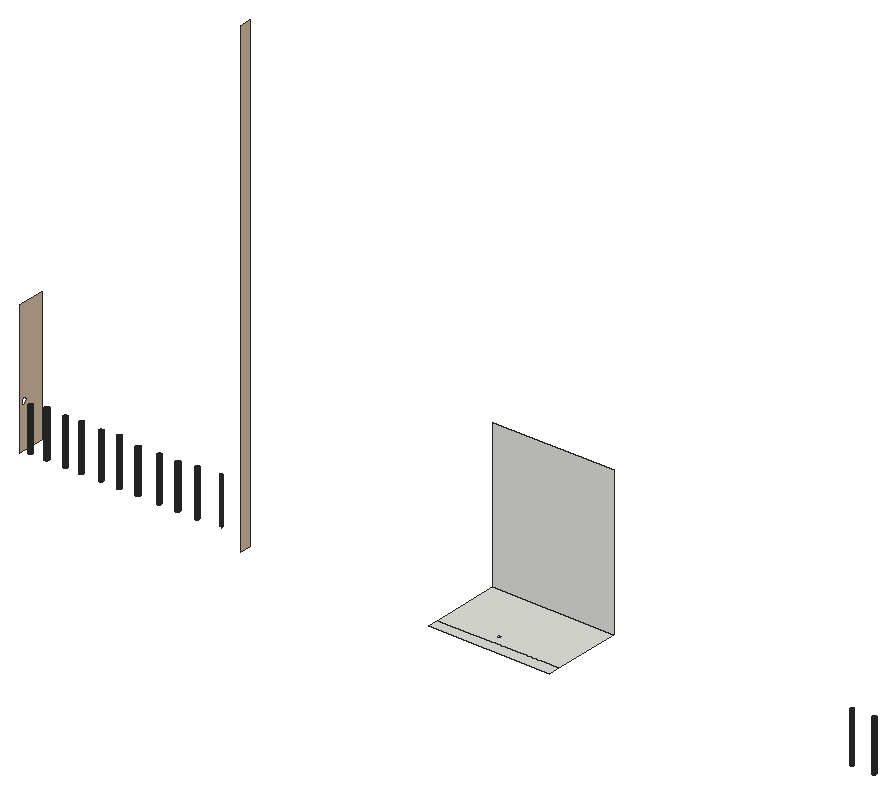
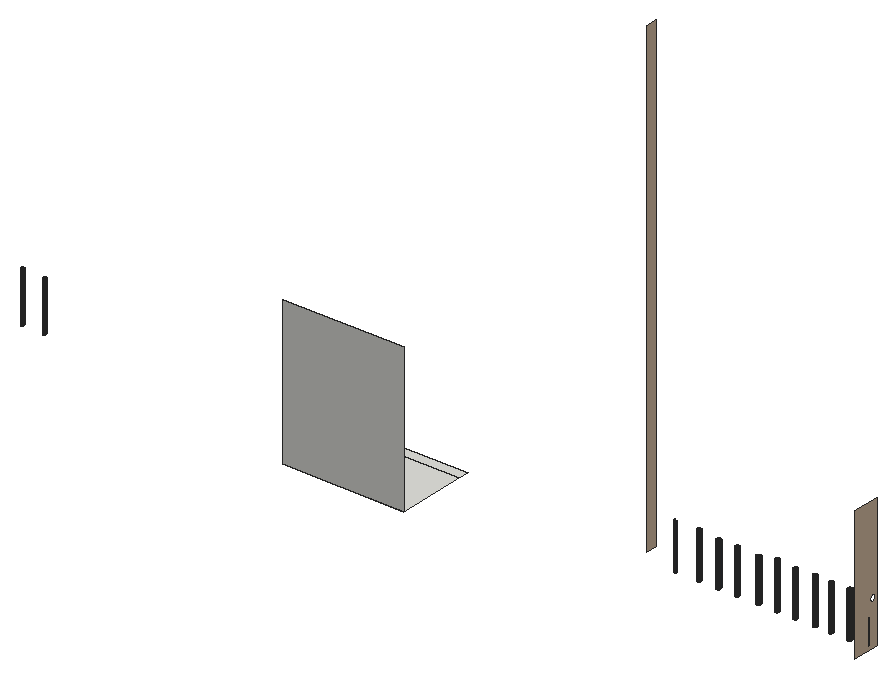
# SketchUp Ruby script. Lengths in inches.
U = 1.inch
M = Sketchup.active_model
def pt(a) = Geom::Point3d.new(a.map { |v| v * U })
def face(e, loops, mat)
  f = e.add_face(loops[0].map { |a| pt(a) })
  loops[1..].each { |l| e.add_face(l.map { |a| pt(a) }).erase! }
  f.material = f.back_material = mat if mat
  f
end
# faces: each face lists its corners as indices into pts; further lists are holes
def faces(e, pts, list, mat = nil) = list.each { |f| face(e, (f[0].is_a?(Array) ? f : [f]).map { |l| l.map { |i| pts[i] } }, mat) }
# xy, xz, yz: faces in a plane at the given z, y or x. An outline is a flat list of corners, or four numbers for a rectangle; further outlines are holes
def ring(l) = l.size == 4 ? [[l[0], l[1]], [l[2], l[1]], [l[2], l[3]], [l[0], l[3]]] : l.each_slice(2).to_a
def flat(e, list, mat, &to3) = list.each { |f| face(e, (f[0].is_a?(Array) ? f : [f]).map { |l| ring(l).map { |u, v| to3.(u, v) } }, mat) }
def xy(e, z, list, mat = nil) = flat(e, list, mat) { |x, y| [x, y, z] }
def xz(e, y, list, mat = nil) = flat(e, list, mat) { |x, z| [x, y, z] }
def yz(e, x, list, mat = nil) = flat(e, list, mat) { |y, z| [x, y, z] }
def lines(e, pts, list) = list.each { |a, b| e.add_line(pt(pts[a]), pt(pts[b])) }
# prism: a flat outline (further loops are holes) pulled along v
def prism(e, loops, v, mat = nil)
  f = face(e, loops, mat); d = Geom::Vector3d.new(v.map { |x| x * U })
  f.pushpull(f.normal.samedirection?(d) ? d.length : -d.length)
end
def box(e, o, s, mat = nil) = prism(e, [[o, [o[0] + s[0], o[1], o[2]], [o[0] + s[0], o[1] + s[1], o[2]], [o[0], o[1] + s[1], o[2]]]], [0, 0, s[2]], mat)
def at(x, y, z, deg = 0) = Geom::Transformation.translation(pt([x, y, z])) * Geom::Transformation.rotation(ORIGIN, Z_AXIS, deg.degrees)
def axes(o, x, y, z) = Geom::Transformation.new([*x, 0, *y, 0, *z, 0, *pt(o).to_a, 1])
def part(name) = M.definitions.add(name)
# library, detail: a bought-in or finely detailed component or shape, given as its bounding box
def library(name, o, s) = part(name).tap { |d| box(d.entities, o, s) }
def detail(e, o, s) = box(e.add_group.entities, o, s)
def put(e, d, t, mat = nil) = e.add_instance(d, t).tap { |i| i.material = mat if mat }
def group(e, t, mat = nil) = e.add_group.tap { |g| g.transformation = t; g.material = mat if mat }.entities
root = M.entities
M.materials.add("[Formica Laminate Dark]").color = [50, 53, 60]
M.materials.add("[Formica Laminate Light]").color = [213, 189, 164]
xy(root,261,[[351.88,110.07,450.54,119.07],[[351.88,119.07,450.54,174.4375],[395.34,125.42,394.9,125.48,394.49,125.65,394.14,125.92,393.875,126.27,393.71,126.67,393.65,127.11,393.71,127.55,393.875,127.95,394.14,128.3,394.49,128.57,394.9,128.74,395.34,128.8,395.77,128.74,396.18,128.57,396.53,128.3,396.8,127.95,396.97,127.55,397.02,127.11,396.97,126.67,396.8,126.27,396.53,125.92,396.18,125.65,395.77,125.48]],[674.41,135.92,674.07,135.96,673.75,136.09,673.48,136.3,673.27,136.57,673.14,136.89,673.1,137.23,673.14,137.57,673.27,137.88,673.48,138.16,673.75,138.36,674.07,138.5,674.41,138.54,674.75,138.5,675.07,138.36,675.34,138.16,675.55,137.88,675.68,137.57,675.72,137.23,675.68,136.89,675.55,136.57,675.34,136.3,675.07,136.09,674.75,135.96],[692.47,135.92,692.13,135.96,691.82,136.09,691.55,136.3,691.34,136.57,691.21,136.89,691.16,137.23,691.21,137.57,691.34,137.88,691.55,138.16,691.82,138.36,692.13,138.5,692.47,138.54,692.8125,138.5,693.13,138.36,693.4,138.16,693.61,137.88,693.74,137.57,693.79,137.23,693.74,136.89,693.61,136.57,693.4,136.3,693.13,136.09,692.8125,135.96]])
xz(root,174.4375,[[351.88,261,450.54,381]])
yz(root,9,[[[122.79,261,144.21,369],[126.49,294.81,125.8,294.9,125.15,295.17,124.59,295.59,124.17,296.15,123.9,296.8,123.81,297.49,123.9,298.1875,124.17,298.84,124.59,299.39,125.15,299.82,125.8,300.09,126.49,300.18,127.1875,300.09,127.84,299.82,128.39,299.39,128.82,298.84,129.09,298.1875,129.18,297.49,129.09,296.8,128.82,296.15,128.39,295.59,127.84,295.17,127.1875,294.9]]],"[Formica Laminate Light]")
yz(root,198.57,[[110.07,261,119.07,645]],"[Formica Laminate Light]")
p = [[13.4,125.48,261],[13.84,125.42,261],[13.84,125.42,295.875],[13.4,125.48,295.875],[14.27,125.48,261],[14.27,125.48,295.875],
  [26.65,125.48,261],[27.09,125.42,261],[27.09,125.42,298.1875],[26.65,125.48,298.1875],[27.52,125.48,261],[27.52,125.48,298.1875],
  [41.96,125.48,261],[42.4,125.42,261],[42.4,125.42,297.49],[41.96,125.48,297.49],[42.84,125.48,261],[42.84,125.48,297.49],
  [54.96,125.48,261],[55.4,125.42,261],[55.4,125.42,298.1875],[54.96,125.48,298.1875],[55.84,125.48,261],[55.84,125.48,298.1875],
  [70.84,125.48,261],[71.27,125.42,261],[71.27,125.42,297.375],[70.84,125.48,297.375],[71.71,125.48,261],[71.71,125.48,297.375],
  [85.78,125.48,261],[86.21,125.42,261],[86.21,125.42,298.84],[85.78,125.48,298.84],[86.65,125.48,261],[86.65,125.48,298.84],
  [100.84,125.48,261],[101.27,125.42,261],[101.27,125.42,296.125],[100.84,125.48,296.125],[101.71,125.48,261],[101.71,125.48,296.125],
  [118.34,125.48,261],[118.77,125.42,261],[118.77,125.42,296.625],[118.34,125.48,296.625],[119.21,125.48,261],[119.21,125.48,296.625],
  [133.4,125.48,261],[133.84,125.42,261],[133.84,125.42,296.5],[133.4,125.48,296.5],[134.27,125.48,261],[134.27,125.48,296.5],
  [149.4,125.48,261],[149.84,125.42,261],[149.84,125.42,298.1875],[149.4,125.48,298.1875],[150.27,125.48,261],[150.27,125.48,298.1875],
  [12.99,125.65,261],[12.99,125.65,295.875],[14.68,125.65,261],[14.68,125.65,295.875],[26.24,125.65,261],[26.24,125.65,298.1875],
  [27.93,125.65,261],[27.93,125.65,298.1875],[41.56,125.65,261],[41.56,125.65,297.49],[43.24,125.65,261],[43.24,125.65,297.49],
  [54.56,125.65,261],[54.56,125.65,298.1875],[56.24,125.65,261],[56.24,125.65,298.1875],[70.43,125.65,261],[70.43,125.65,297.375],
  [72.12,125.65,261],[72.12,125.65,297.375],[85.37,125.65,261],[85.37,125.65,298.84],[87.06,125.65,261],[87.06,125.65,298.84],
  [100.43,125.65,261],[100.43,125.65,296.125],[102.12,125.65,261],[102.12,125.65,296.125],[117.93,125.65,261],[117.93,125.65,296.625],
  [119.62,125.65,261],[119.62,125.65,296.625],[132.99,125.65,261],[132.99,125.65,296.5],[134.68,125.65,261],[134.68,125.65,296.5],
  [148.99,125.65,261],[148.99,125.65,298.1875],[150.68,125.65,261],[150.68,125.65,298.1875],[12.64,125.92,261],[12.64,125.92,295.875],
  [15.03,125.92,261],[15.03,125.92,295.875],[25.89,125.92,261],[25.89,125.92,298.1875],[28.28,125.92,261],[28.28,125.92,298.1875],
  [41.21,125.92,261],[41.21,125.92,297.49],[43.59,125.92,261],[43.59,125.92,297.49],[54.21,125.92,261],[54.21,125.92,298.1875],
  [56.59,125.92,261],[56.59,125.92,298.1875],[70.08,125.92,261],[70.08,125.92,297.375],[72.47,125.92,261],[72.47,125.92,297.375],
  [85.02,125.92,261],[85.02,125.92,298.84],[87.41,125.92,261],[87.41,125.92,298.84],[100.08,125.92,261],[100.08,125.92,296.125],
  [102.47,125.92,261],[102.47,125.92,296.125],[117.58,125.92,261],[117.58,125.92,296.625],[119.97,125.92,261],[119.97,125.92,296.625],
  [132.64,125.92,261],[132.64,125.92,296.5],[135.03,125.92,261],[135.03,125.92,296.5],[148.64,125.92,261],[148.64,125.92,298.1875],
  [151.03,125.92,261],[151.03,125.92,298.1875],[12.375,126.27,261],[12.375,126.27,295.875],[15.3,126.27,261],[15.3,126.27,295.875],
  [25.625,126.27,261],[25.625,126.27,298.1875],[28.55,126.27,261],[28.55,126.27,298.1875],[40.9375,126.27,261],[40.9375,126.27,297.49],
  [43.86,126.27,261],[43.86,126.27,297.49],[53.9375,126.27,261],[53.9375,126.27,298.1875],[56.86,126.27,261],[56.86,126.27,298.1875],
  [69.8125,126.27,261],[69.8125,126.27,297.375],[72.74,126.27,261],[72.74,126.27,297.375],[84.75,126.27,261],[84.75,126.27,298.84],
  [87.67,126.27,261],[87.67,126.27,298.84],[99.8125,126.27,261],[99.8125,126.27,296.125],[102.74,126.27,261],[102.74,126.27,296.125],
  [117.3125,126.27,261],[117.3125,126.27,296.625],[120.24,126.27,261],[120.24,126.27,296.625],[132.375,126.27,261],[132.375,126.27,296.5],
  [135.3,126.27,261],[135.3,126.27,296.5],[148.375,126.27,261],[148.375,126.27,298.1875],[151.3,126.27,261],[151.3,126.27,298.1875],
  [12.21,126.67,261],[12.21,126.67,295.875],[15.47,126.67,261],[15.47,126.67,295.875],[25.46,126.67,261],[25.46,126.67,298.1875],
  [28.72,126.67,261],[28.72,126.67,298.1875],[40.77,126.67,261],[40.77,126.67,297.49],[44.03,126.67,261],[44.03,126.67,297.49],
  [53.77,126.67,261],[53.77,126.67,298.1875],[57.03,126.67,261],[57.03,126.67,298.1875],[69.64,126.67,261],[69.64,126.67,297.375],
  [72.9,126.67,261],[72.9,126.67,297.375],[84.58,126.67,261],[84.58,126.67,298.84],[87.84,126.67,261],[87.84,126.67,298.84],
  [99.64,126.67,261],[99.64,126.67,296.125],[102.9,126.67,261],[102.9,126.67,296.125],[117.14,126.67,261],[117.14,126.67,296.625],
  [120.4,126.67,261],[120.4,126.67,296.625],[132.21,126.67,261],[132.21,126.67,296.5],[135.47,126.67,261],[135.47,126.67,296.5],
  [148.21,126.67,261],[148.21,126.67,298.1875],[151.47,126.67,261],[151.47,126.67,298.1875],[12.15,127.11,261],[12.15,127.11,295.875],
  [15.52,127.11,261],[15.52,127.11,295.875],[25.4,127.11,261],[25.4,127.11,298.1875],[28.77,127.11,261],[28.77,127.11,298.1875],
  [40.71,127.11,261],[40.71,127.11,297.49],[44.09,127.11,261],[44.09,127.11,297.49],[53.71,127.11,261],[53.71,127.11,298.1875],
  [57.09,127.11,261],[57.09,127.11,298.1875],[69.59,127.11,261],[69.59,127.11,297.375],[72.96,127.11,261],[72.96,127.11,297.375],
  [84.52,127.11,261],[84.52,127.11,298.84],[87.9,127.11,261],[87.9,127.11,298.84],[99.59,127.11,261],[99.59,127.11,296.125],
  [102.96,127.11,261],[102.96,127.11,296.125],[117.09,127.11,261],[117.09,127.11,296.625],[120.46,127.11,261],[120.46,127.11,296.625],
  [132.15,127.11,261],[132.15,127.11,296.5],[135.52,127.11,261],[135.52,127.11,296.5],[148.15,127.11,261],[148.15,127.11,298.1875],
  [151.52,127.11,261],[151.52,127.11,298.1875],[169.59,126.67,261],[169.65,127.11,261],[169.65,127.11,298.84],[169.59,126.67,298.84],
  [12.21,127.55,261],[12.21,127.55,295.875],[15.47,127.55,261],[15.47,127.55,295.875],[25.46,127.55,261],[25.46,127.55,298.1875],
  [28.72,127.55,261],[28.72,127.55,298.1875],[40.77,127.55,261],[40.77,127.55,297.49],[44.03,127.55,261],[44.03,127.55,297.49],
  [53.77,127.55,261],[53.77,127.55,298.1875],[57.03,127.55,261],[57.03,127.55,298.1875],[69.64,127.55,261],[69.64,127.55,297.375],
  [72.9,127.55,261],[72.9,127.55,297.375],[84.58,127.55,261],[84.58,127.55,298.84],[87.84,127.55,261],[87.84,127.55,298.84],
  [99.64,127.55,261],[99.64,127.55,296.125],[102.9,127.55,261],[102.9,127.55,296.125],[117.14,127.55,261],[117.14,127.55,296.625],
  [120.4,127.55,261],[120.4,127.55,296.625],[132.21,127.55,261],[132.21,127.55,296.5],[135.47,127.55,261],[135.47,127.55,296.5],
  [148.21,127.55,261],[148.21,127.55,298.1875],[151.47,127.55,261],[151.47,127.55,298.1875],[169.59,127.55,261],[169.59,127.55,298.84],
  [12.375,127.95,261],[12.375,127.95,295.875],[15.3,127.95,261],[15.3,127.95,295.875],[25.625,127.95,261],[25.625,127.95,298.1875],
  [28.55,127.95,261],[28.55,127.95,298.1875],[40.9375,127.95,261],[40.9375,127.95,297.49],[43.86,127.95,261],[43.86,127.95,297.49],
  [53.9375,127.95,261],[53.9375,127.95,298.1875],[56.86,127.95,261],[56.86,127.95,298.1875],[69.8125,127.95,261],[69.8125,127.95,297.375],
  [72.74,127.95,261],[72.74,127.95,297.375],[84.75,127.95,261],[84.75,127.95,298.84],[87.67,127.95,261],[87.67,127.95,298.84],
  [99.8125,127.95,261],[99.8125,127.95,296.125],[102.74,127.95,261],[102.74,127.95,296.125],[117.3125,127.95,261],[117.3125,127.95,296.625],
  [120.24,127.95,261],[120.24,127.95,296.625],[132.375,127.95,261],[132.375,127.95,296.5],[135.3,127.95,261],[135.3,127.95,296.5],
  [148.375,127.95,261],[148.375,127.95,298.1875],[151.3,127.95,261],[151.3,127.95,298.1875],[169.42,127.95,261],[169.42,127.95,298.84],
  [12.64,128.3,261],[12.64,128.3,295.875],[15.03,128.3,261],[15.03,128.3,295.875],[25.89,128.3,261],[25.89,128.3,298.1875],
  [28.28,128.3,261],[28.28,128.3,298.1875],[41.21,128.3,261],[41.21,128.3,297.49],[43.59,128.3,261],[43.59,128.3,297.49],
  [54.21,128.3,261],[54.21,128.3,298.1875],[56.59,128.3,261],[56.59,128.3,298.1875],[70.08,128.3,261],[70.08,128.3,297.375],
  [72.47,128.3,261],[72.47,128.3,297.375],[85.02,128.3,261],[85.02,128.3,298.84],[87.41,128.3,261],[87.41,128.3,298.84],
  [100.08,128.3,261],[100.08,128.3,296.125],[102.47,128.3,261],[102.47,128.3,296.125],[117.58,128.3,261],[117.58,128.3,296.625],
  [119.97,128.3,261],[119.97,128.3,296.625],[132.64,128.3,261],[132.64,128.3,296.5],[135.03,128.3,261],[135.03,128.3,296.5],
  [148.64,128.3,261],[148.64,128.3,298.1875],[151.03,128.3,261],[151.03,128.3,298.1875],[169.16,128.3,261],[169.16,128.3,298.84],
  [12.99,128.57,261],[12.99,128.57,295.875],[14.68,128.57,261],[14.68,128.57,295.875],[26.24,128.57,261],[26.24,128.57,298.1875],
  [27.93,128.57,261],[27.93,128.57,298.1875],[41.56,128.57,261],[41.56,128.57,297.49],[43.24,128.57,261],[43.24,128.57,297.49],
  [54.56,128.57,261],[54.56,128.57,298.1875],[56.24,128.57,261],[56.24,128.57,298.1875],[70.43,128.57,261],[70.43,128.57,297.375],
  [72.12,128.57,261],[72.12,128.57,297.375],[85.37,128.57,261],[85.37,128.57,298.84],[87.06,128.57,261],[87.06,128.57,298.84],
  [100.43,128.57,261],[100.43,128.57,296.125],[102.12,128.57,261],[102.12,128.57,296.125],[117.93,128.57,261],[117.93,128.57,296.625],
  [119.62,128.57,261],[119.62,128.57,296.625],[132.99,128.57,261],[132.99,128.57,296.5],[134.68,128.57,261],[134.68,128.57,296.5],
  [148.99,128.57,261],[148.99,128.57,298.1875],[150.68,128.57,261],[150.68,128.57,298.1875],[168.81,128.57,261],[168.81,128.57,298.84],
  [13.4,128.74,261],[13.4,128.74,295.875],[14.27,128.74,261],[14.27,128.74,295.875],[26.65,128.74,261],[26.65,128.74,298.1875],
  [27.52,128.74,261],[27.52,128.74,298.1875],[41.96,128.74,261],[41.96,128.74,297.49],[42.84,128.74,261],[42.84,128.74,297.49],
  [54.96,128.74,261],[54.96,128.74,298.1875],[55.84,128.74,261],[55.84,128.74,298.1875],[70.84,128.74,261],[70.84,128.74,297.375],
  [71.71,128.74,261],[71.71,128.74,297.375],[85.78,128.74,261],[85.78,128.74,298.84],[86.65,128.74,261],[86.65,128.74,298.84],
  [100.84,128.74,261],[100.84,128.74,296.125],[101.71,128.74,261],[101.71,128.74,296.125],[118.34,128.74,261],[118.34,128.74,296.625],
  [119.21,128.74,261],[119.21,128.74,296.625],[133.4,128.74,261],[133.4,128.74,296.5],[134.27,128.74,261],[134.27,128.74,296.5],
  [149.4,128.74,261],[149.4,128.74,298.1875],[150.27,128.74,261],[150.27,128.74,298.1875],[167.53,128.74,261],[167.12,128.57,261],
  [167.12,128.57,298.84],[167.53,128.74,298.84],[168.4,128.74,261],[168.4,128.74,298.84],[13.84,128.8,261],[13.84,128.8,295.875],
  [27.09,128.8,261],[27.09,128.8,298.1875],[42.4,128.8,261],[42.4,128.8,297.49],[55.4,128.8,261],[55.4,128.8,298.1875],
  [71.27,128.8,261],[71.27,128.8,297.375],[86.21,128.8,261],[86.21,128.8,298.84],[101.27,128.8,261],[101.27,128.8,296.125],
  [118.77,128.8,261],[118.77,128.8,296.625],[133.84,128.8,261],[133.84,128.8,296.5],[149.84,128.8,261],[149.84,128.8,298.1875],
  [167.96,128.8,261],[167.96,128.8,298.84],[674.07,135.96,261],[674.41,135.92,261],[674.41,135.92,301.75],[674.07,135.96,301.75],
  [674.75,135.96,261],[674.75,135.96,301.75],[692.13,135.96,261],[692.47,135.92,261],[692.47,135.92,302.51],[692.13,135.96,302.51],
  [692.8125,135.96,261],[692.8125,135.96,302.51],[673.75,136.09,261],[673.75,136.09,301.75],[675.07,136.09,261],[675.07,136.09,301.75],
  [691.82,136.09,261],[691.82,136.09,302.51],[693.13,136.09,261],[693.13,136.09,302.51],[673.48,136.3,261],[673.48,136.3,301.75],
  [675.34,136.3,261],[675.34,136.3,301.75],[691.55,136.3,261],[691.55,136.3,302.51],[693.4,136.3,261],[693.4,136.3,302.51],
  [673.27,136.57,261],[673.27,136.57,301.75],[675.55,136.57,261],[675.55,136.57,301.75],[691.34,136.57,261],[691.34,136.57,302.51],
  [693.61,136.57,261],[693.61,136.57,302.51],[673.14,136.89,261],[673.14,136.89,301.75],[675.68,136.89,261],[675.68,136.89,301.75],
  [691.21,136.89,261],[691.21,136.89,302.51],[693.74,136.89,261],[693.74,136.89,302.51],[673.1,137.23,261],[673.1,137.23,301.75],
  [675.72,137.23,261],[675.72,137.23,301.75],[691.16,137.23,261],[691.18,137.06,302.51],[691.16,137.23,302.51],[693.79,137.23,261],
  [693.79,137.23,302.51],[693.76,137.06,302.51],[673.14,137.57,261],[673.14,137.57,301.75],[675.68,137.57,261],[675.68,137.57,301.75],
  [691.21,137.57,261],[691.21,137.57,302.51],[693.74,137.57,261],[693.74,137.57,302.51],[673.27,137.88,261],[673.27,137.88,301.75],
  [675.55,137.88,261],[675.55,137.88,301.75],[691.34,137.88,261],[691.34,137.88,302.51],[693.61,137.88,261],[693.61,137.88,302.51],
  [673.48,138.16,261],[673.48,138.16,301.75],[675.34,138.16,261],[675.34,138.16,301.75],[691.55,138.16,261],[691.55,138.16,302.51],
  [693.4,138.16,261],[693.4,138.16,302.51],[673.75,138.36,261],[673.75,138.36,301.75],[675.07,138.36,261],[675.07,138.36,301.75],
  [691.82,138.36,261],[691.82,138.36,302.51],[693.13,138.36,261],[693.13,138.36,302.51],[674.07,138.5,261],[674.07,138.5,301.75],
  [674.75,138.5,261],[674.75,138.5,301.75],[692.13,138.5,261],[692.13,138.5,302.51],[692.8125,138.5,261],[692.8125,138.5,302.51],
  [674.41,138.54,261],[674.41,138.54,301.75],[692.47,138.54,261],[692.47,138.54,302.51]]
faces(root,p,[[0,1,2,3],[1,4,5,2],[6,7,8,9],[7,10,11,8],[12,13,14,15],[13,16,17,14],[18,19,20,21],[19,22,23,20],
  [24,25,26,27],[25,28,29,26],[30,31,32,33],[31,34,35,32],[36,37,38,39],[37,40,41,38],[42,43,44,45],[43,46,47,44],
  [48,49,50,51],[49,52,53,50],[54,55,56,57],[55,58,59,56],[60,0,3,61],[4,62,63,5],[64,6,9,65],[10,66,67,11],
  [68,12,15,69],[16,70,71,17],[72,18,21,73],[22,74,75,23],[76,24,27,77],[28,78,79,29],[80,30,33,81],[34,82,83,35],
  [84,36,39,85],[40,86,87,41],[88,42,45,89],[46,90,91,47],[92,48,51,93],[52,94,95,53],[96,54,57,97],[58,98,99,59],
  [100,60,61,101],[62,102,103,63],[104,64,65,105],[66,106,107,67],[108,68,69,109],[70,110,111,71],[112,72,73,113],[74,114,115,75],
  [116,76,77,117],[78,118,119,79],[120,80,81,121],[82,122,123,83],[124,84,85,125],[86,126,127,87],[128,88,89,129],[90,130,131,91],
  [132,92,93,133],[94,134,135,95],[136,96,97,137],[98,138,139,99],[140,100,101,141],[102,142,143,103],[144,104,105,145],[106,146,147,107],
  [148,108,109,149],[110,150,151,111],[152,112,113,153],[114,154,155,115],[156,116,117,157],[118,158,159,119],[160,120,121,161],[122,162,163,123],
  [164,124,125,165],[126,166,167,127],[168,128,129,169],[130,170,171,131],[172,132,133,173],[134,174,175,135],[176,136,137,177],[138,178,179,139],
  [180,140,141,181],[142,182,183,143],[184,144,145,185],[146,186,187,147],[188,148,149,189],[150,190,191,151],[192,152,153,193],[154,194,195,155],
  [196,156,157,197],[158,198,199,159],[200,160,161,201],[162,202,203,163],[204,164,165,205],[166,206,207,167],[208,168,169,209],[170,210,211,171],
  [212,172,173,213],[174,214,215,175],[216,176,177,217],[178,218,219,179],[220,180,181,221],[182,222,223,183],[224,184,185,225],[186,226,227,187],
  [228,188,189,229],[190,230,231,191],[232,192,193,233],[194,234,235,195],[236,196,197,237],[198,238,239,199],[240,200,201,241],[202,242,243,203],
  [244,204,205,245],[206,246,247,207],[248,208,209,249],[210,250,251,211],[252,212,213,253],[214,254,255,215],[256,216,217,257],[218,258,259,219],
  [260,261,262,263],[264,220,221,265],[222,266,267,223],[268,224,225,269],[226,270,271,227],[272,228,229,273],[230,274,275,231],[276,232,233,277],
  [234,278,279,235],[280,236,237,281],[238,282,283,239],[284,240,241,285],[242,286,287,243],[288,244,245,289],[246,290,291,247],[292,248,249,293],
  [250,294,295,251],[296,252,253,297],[254,298,299,255],[300,256,257,301],[258,302,303,259],[261,304,305,262],[306,264,265,307],[266,308,309,267],
  [310,268,269,311],[270,312,313,271],[314,272,273,315],[274,316,317,275],[318,276,277,319],[278,320,321,279],[322,280,281,323],[282,324,325,283],
  [326,284,285,327],[286,328,329,287],[330,288,289,331],[290,332,333,291],[334,292,293,335],[294,336,337,295],[338,296,297,339],[298,340,341,299],
  [342,300,301,343],[302,344,345,303],[304,346,347,305],[348,306,307,349],[308,350,351,309],[352,310,311,353],[312,354,355,313],[356,314,315,357],
  [316,358,359,317],[360,318,319,361],[320,362,363,321],[364,322,323,365],[324,366,367,325],[368,326,327,369],[328,370,371,329],[372,330,331,373],
  [332,374,375,333],[376,334,335,377],[336,378,379,337],[380,338,339,381],[340,382,383,341],[384,342,343,385],[344,386,387,345],[346,388,389,347],
  [390,348,349,391],[350,392,393,351],[394,352,353,395],[354,396,397,355],[398,356,357,399],[358,400,401,359],[402,360,361,403],[362,404,405,363],
  [406,364,365,407],[366,408,409,367],[410,368,369,411],[370,412,413,371],[414,372,373,415],[374,416,417,375],[418,376,377,419],[378,420,421,379],
  [422,380,381,423],[382,424,425,383],[426,384,385,427],[386,428,429,387],[388,430,431,389],[432,390,391,433],[392,434,435,393],[436,394,395,437],
  [396,438,439,397],[440,398,399,441],[400,442,443,401],[444,402,403,445],[404,446,447,405],[448,406,407,449],[408,450,451,409],[452,410,411,453],
  [412,454,455,413],[456,414,415,457],[416,458,459,417],[460,418,419,461],[420,462,463,421],[464,422,423,465],[424,466,467,425],[468,426,427,469],
  [428,470,471,429],[472,473,474,475],[430,476,477,431],[478,432,433,479],[434,478,479,435],[480,436,437,481],[438,480,481,439],[482,440,441,483],
  [442,482,483,443],[484,444,445,485],[446,484,485,447],[486,448,449,487],[450,486,487,451],[488,452,453,489],[454,488,489,455],[490,456,457,491],
  [458,490,491,459],[492,460,461,493],[462,492,493,463],[494,464,465,495],[466,494,495,467],[496,468,469,497],[470,496,497,471],[498,472,475,499],
  [476,498,499,477],[500,501,502,503],[501,504,505,502],[506,507,508,509],[507,510,511,508],[512,500,503,513],[504,514,515,505],[516,506,509,517],
  [510,518,519,511],[520,512,513,521],[514,522,523,515],[524,516,517,525],[518,526,527,519],[528,520,521,529],[522,530,531,523],[532,524,525,533],
  [526,534,535,527],[536,528,529,537],[530,538,539,531],[540,532,533,541],[534,542,543,535],[544,536,537,545],[538,546,547,539],[548,540,541,549,550],
  [542,551,552,553,543],[554,544,545,555],[546,556,557,547],[558,548,550,559],[551,560,561,552],[562,554,555,563],[556,564,565,557],[566,558,559,567],
  [560,568,569,561],[570,562,563,571],[564,572,573,565],[574,566,567,575],[568,576,577,569],[578,570,571,579],[572,580,581,573],[582,574,575,583],
  [576,584,585,577],[586,578,579,587],[580,588,589,581],[590,582,583,591],[584,592,593,585],[594,586,587,595],[588,594,595,589],[596,590,591,597],
  [592,596,597,593]],"[Formica Laminate Dark]")
